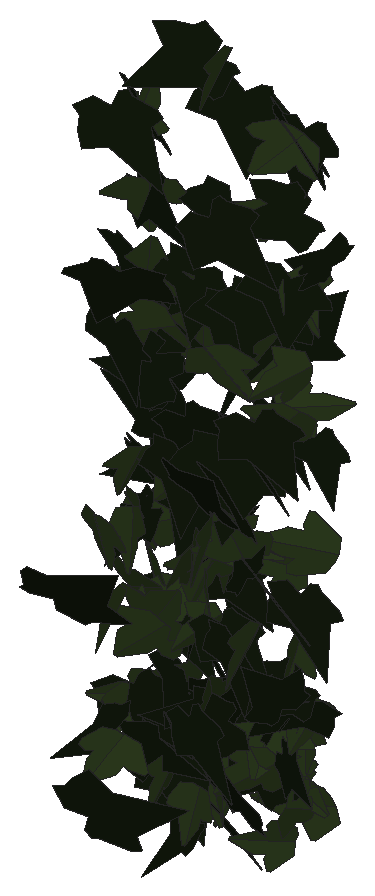
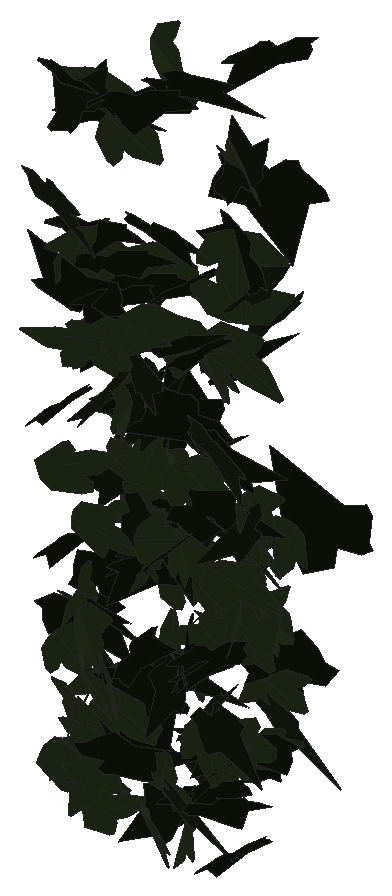
# SketchUp Ruby script. Lengths in inches.
U = 1.inch
M = Sketchup.active_model
def pt(a) = Geom::Point3d.new(a.map { |v| v * U })
def face(e, loops, mat)
  f = e.add_face(loops[0].map { |a| pt(a) })
  loops[1..].each { |l| e.add_face(l.map { |a| pt(a) }).erase! }
  f.material = f.back_material = mat if mat
  f
end
# faces: each face lists its corners as indices into pts; further lists are holes
def faces(e, pts, list, mat = nil) = list.each { |f| face(e, (f[0].is_a?(Array) ? f : [f]).map { |l| l.map { |i| pts[i] } }, mat) }
# xy, xz, yz: faces in a plane at the given z, y or x. An outline is a flat list of corners, or four numbers for a rectangle; further outlines are holes
def ring(l) = l.size == 4 ? [[l[0], l[1]], [l[2], l[1]], [l[2], l[3]], [l[0], l[3]]] : l.each_slice(2).to_a
def flat(e, list, mat, &to3) = list.each { |f| face(e, (f[0].is_a?(Array) ? f : [f]).map { |l| ring(l).map { |u, v| to3.(u, v) } }, mat) }
def xy(e, z, list, mat = nil) = flat(e, list, mat) { |x, y| [x, y, z] }
def xz(e, y, list, mat = nil) = flat(e, list, mat) { |x, z| [x, y, z] }
def yz(e, x, list, mat = nil) = flat(e, list, mat) { |y, z| [x, y, z] }
def lines(e, pts, list) = list.each { |a, b| e.add_line(pt(pts[a]), pt(pts[b])) }
# prism: a flat outline (further loops are holes) pulled along v
def prism(e, loops, v, mat = nil)
  f = face(e, loops, mat); d = Geom::Vector3d.new(v.map { |x| x * U })
  f.pushpull(f.normal.samedirection?(d) ? d.length : -d.length)
end
def box(e, o, s, mat = nil) = prism(e, [[o, [o[0] + s[0], o[1], o[2]], [o[0] + s[0], o[1] + s[1], o[2]], [o[0], o[1] + s[1], o[2]]]], [0, 0, s[2]], mat)
def at(x, y, z, deg = 0) = Geom::Transformation.translation(pt([x, y, z])) * Geom::Transformation.rotation(ORIGIN, Z_AXIS, deg.degrees)
def axes(o, x, y, z) = Geom::Transformation.new([*x, 0, *y, 0, *z, 0, *pt(o).to_a, 1])
def part(name) = M.definitions.add(name)
# library, detail: a bought-in or finely detailed component or shape, given as its bounding box
def library(name, o, s) = part(name).tap { |d| box(d.entities, o, s) }
def detail(e, o, s) = box(e.add_group.entities, o, s)
def put(e, d, t, mat = nil) = e.add_instance(d, t).tap { |i| i.material = mat if mat }
def group(e, t, mat = nil) = e.add_group.tap { |g| g.transformation = t; g.material = mat if mat }.entities
root = M.entities
M.materials.add("1026 AP 7946 SUNNY SIDE UP").color = [254, 231, 186]
M.materials.add("efeu1").color = [18, 25, 13]
M.materials.add("efeu2").color = [43, 57, 29]
c1 = part("ivyleaf_9")
p = [[1.54,2.16,1.25],[1.36,2.04,1.19],[-0.21,0.99,0.68],[-0.71,1.11,0.82],[-0.85,0.86,0.67],[-0.8,0.17,0.21],
  [-0.9,-0.01,0.1],[-0.67,-0.16,-0.02],[-0.08,-0.08,-0.05],[-0.03,-0.6,-0.4],[0.65,-0.88,-0.66],[0.83,-0.6,-0.49],
  [1.29,-0.42,-0.43],[1.8125,-0.07,-0.26],[1.21,0.44,0.15]]
faces(c1.entities,p,[[0,1,2,3,4,5,6,7,8,9,10,11,12,13,14]],"efeu1")
c2 = part("ivyleaf_10")
p = [[0,0.5,-0.03],[-0.0625,2.02,-0.43],[-0.19,2.01,-0.46],[-0.54,1.05,-0.29],[-0.52,0.625,-0.18],[-0.83,0.76,-0.28],
  [-1.16,0.64,-0.33],[-1.15,0.33,-0.24],[-0.77,-0.39,0.02],[-0.3,-0.51,0.16],[0.04,-0.48,0.23],[-0.02,2.01,-0.4375],
  [-0.06,2.01,-0.43],[0.04,-0.49,0.23],[0.67,-0.49,0.14],[1.38,0.36,-0.2],[1.375,0.51,-0.24],[0.81,0.65,-0.19],
  [0.62,0.59,-0.15],[0.6,1.09,-0.28],[0.5,1.23,-0.31]]
faces(c2.entities,p,[[0,1,2,3,4,5,6,7,8,9,10],[11,12,0,13,14,15,16,17,18,19,20]],"efeu2")
put(root,c1,axes([122.75,208.77,268.89],[0.03474,0.02424,0.377],[0.53606,-0.13615,-0.01271],[0.21202,0.34025,-0.02963]),"1026 AP 7946 SUNNY SIDE UP")
put(root,c1,axes([121.66,209.41,271.47],[0.60179,0.0809,-0.03944],[0.04372,0.05444,0.40035],[0.1341,-0.38081,0.04648]),"1026 AP 7946 SUNNY SIDE UP")
put(root,c2,axes([123.75,209.64,269.13],[0.39833,-0.15611,0.07489],[0.07791,-0.05941,-0.3059],[0.25994,0.25702,-0.02308]),"1026 AP 7946 SUNNY SIDE UP")
put(root,c2,axes([122.36,209.76,269.38],[0.30396,0.15864,-0.17189],[-0.1758,-0.12711,-0.2573],[-0.31765,0.22216,-0.02208]),"1026 AP 7946 SUNNY SIDE UP")
put(root,c1,axes([122.5,209.63,276.52],[0.28706,0.22973,-0.2263],[-0.18683,-0.18725,-0.30277],[-0.46509,0.21701,-0.01805]),"1026 AP 7946 SUNNY SIDE UP")
put(root,c1,axes([123.41,210.02,269.98],[0.19558,-0.3098,-0.09677],[-0.07178,0.08094,-0.34322],[0.50313,0.13197,-0.01135]),"1026 AP 7946 SUNNY SIDE UP")
put(root,c2,axes([124.22,210.21,271.46],[0.09418,-0.28362,0.22119],[0.1015,-0.2071,-0.29937],[0.55161,0.08653,0.01732]),"1026 AP 7946 SUNNY SIDE UP")
put(root,c1,axes([122.08,210.05,278.63],[0.03794,-0.29954,-0.21207],[0.02738,0.20533,-0.30704],[0.56934,0.01009,0.0289]),"1026 AP 7946 SUNNY SIDE UP")
put(root,c1,axes([121.99,210.16,269.31],[-0.37422,0.23918,-0.03857],[0.01295,-0.04637,-0.34678],[-0.38078,-0.23663,0.02612]),"1026 AP 7946 SUNNY SIDE UP")
put(root,c1,axes([123.23,210.27,268.25],[-0.37725,0.13435,-0.15103],[0.16463,-0.11135,-0.28083],[-0.26688,-0.25861,0.04026]),"1026 AP 7946 SUNNY SIDE UP")
put(root,c1,axes([123.67,210.13,277.5],[0.10698,-0.22666,-0.28735],[-0.03255,0.27964,-0.23878],[0.56263,0.05928,0.04082]),"1026 AP 7946 SUNNY SIDE UP")
put(root,c1,axes([123.8,210.43,271.08],[0.02352,-0.30816,0.07438],[0.00007,-0.07403,-0.31825],[0.49831,0.01455,-0.00346]),"1026 AP 7946 SUNNY SIDE UP")
put(root,c2,axes([123.31,210.48,272.58],[0.16811,-0.25804,0.21936],[0.15013,-0.19231,-0.28862],[0.5057,0.14287,0.01277]),"1026 AP 7946 SUNNY SIDE UP")
put(root,c1,axes([123.08,210.46,273.07],[0.49405,-0.12793,-0.06342],[0.1154,0.02041,0.3464],[-0.19052,-0.31938,0.04537]),"1026 AP 7946 SUNNY SIDE UP")
put(root,c1,axes([124.52,210.48,270.39],[0.10657,0.0934,0.29273],[-0.36115,-0.16955,0.11307],[0.30005,-0.23725,0.03212]),"1026 AP 7946 SUNNY SIDE UP")
put(root,c1,axes([121.72,210.57,275.05],[0.07536,-0.34041,0.10363],[0.03011,-0.10083,-0.3547],[0.5582,0.0514,0.00514]),"1026 AP 7946 SUNNY SIDE UP")
put(root,c2,axes([121.71,210.59,270.93],[0.10354,-0.24939,0.23301],[0.12107,-0.21469,-0.26655],[0.51691,0.10024,0.01575]),"1026 AP 7946 SUNNY SIDE UP")
put(root,c1,axes([124.1,210.55,272.1],[0.28603,-0.21039,0.12753],[0.09847,-0.11053,-0.28621],[0.37197,0.19103,-0.0223]),"1026 AP 7946 SUNNY SIDE UP")
put(root,c2,axes([123.47,210.42,275.27],[-0.39701,-0.06742,-0.16391],[0.25675,-0.00295,-0.26632],[0.08722,-0.29822,0.03785]),"1026 AP 7946 SUNNY SIDE UP")
put(root,c1,axes([123.57,210.46,271.27],[0.09627,-0.26634,-0.16801],[0.04134,0.1685,-0.27488],[0.48808,0.03826,0.05642]),"1026 AP 7946 SUNNY SIDE UP")
put(root,c2,axes([121.53,210.45,272.08],[-0.39499,0.15912,-0.01322],[-0.00242,-0.02801,-0.30546],[-0.25111,-0.25001,0.02374]),"1026 AP 7946 SUNNY SIDE UP")
put(root,c2,axes([123.1,210.78,271.05],[-0.04722,-0.11263,0.28485],[0.00635,-0.27867,-0.11785],[0.47035,-0.00755,0.03019]),"1026 AP 7946 SUNNY SIDE UP")
put(root,c2,axes([122.4375,210.74,268.65],[0.02735,-0.23179,0.2053],[0.10044,-0.19377,-0.2375],[0.47142,0.05473,0.03869]),"1026 AP 7946 SUNNY SIDE UP")
put(root,c2,axes([124.51,210.83,275.23],[-0.04906,-0.07801,0.33838],[-0.01486,-0.32997,-0.08348],[0.53131,-0.01643,0.02891]),"1026 AP 7946 SUNNY SIDE UP")
put(root,c2,axes([122.96,210.52,272.14],[0.05841,-0.33956,-0.1479],[0.01997,0.14346,-0.35003],[0.57817,0.02935,0.02703]),"1026 AP 7946 SUNNY SIDE UP")
put(root,c2,axes([123.68,210.68,272.35],[-0.37359,-0.19004,-0.13045],[-0.18168,-0.05578,0.31192],[-0.30864,0.26287,-0.02571]),"1026 AP 7946 SUNNY SIDE UP")
put(root,c2,axes([122.32,210.65,270.69],[-0.37508,-0.07457,0.21036],[-0.27563,-0.11435,-0.25412],[0.20321,-0.29274,0.0436]),"1026 AP 7946 SUNNY SIDE UP")
put(root,c1,axes([123.44,210.67,269.71],[-0.09254,-0.08527,-0.29251],[-0.36862,-0.16301,0.09971],[-0.28415,0.23924,-0.03409]),"1026 AP 7946 SUNNY SIDE UP")
put(root,c1,axes([123.62,210.74,272.9],[0.18318,-0.30368,0.05041],[0.00472,0.05528,0.33461],[-0.48409,-0.11437,0.02234]),"1026 AP 7946 SUNNY SIDE UP")
put(root,c1,axes([121.92,210.58,268.94],[0.17731,-0.03785,-0.27747],[0.3614,0.16876,0.07575],[0.22804,-0.23804,0.0957]),"1026 AP 7946 SUNNY SIDE UP")
put(root,c1,axes([122.3,210.86,274.35],[-0.13919,-0.0046,0.32221],[-0.37911,-0.20612,-0.07462],[0.31341,-0.25137,0.05284]),"1026 AP 7946 SUNNY SIDE UP")
put(root,c1,axes([123.97,210.65,274.31],[-0.07011,-0.23844,-0.23444],[0.0656,0.22234,-0.2486],[0.51263,-0.06106,-0.00025]),"1026 AP 7946 SUNNY SIDE UP")
put(root,c2,axes([121.74,210.8,272.07],[0.35308,-0.15175,0.17713],[0.20708,-0.11313,-0.27932],[0.29644,0.25977,-0.01585]),"1026 AP 7946 SUNNY SIDE UP")
put(root,c2,axes([123.15,210.83,269.9],[-0.07626,-0.24225,-0.17779],[-0.01191,-0.17241,0.25252],[-0.46629,0.04402,0.02263]),"1026 AP 7946 SUNNY SIDE UP")
put(root,c2,axes([122.27,210.6875,270.83],[-0.45804,0.02765,0.14058],[0.21745,0.02403,0.29959],[0.02319,0.32071,-0.03267]),"1026 AP 7946 SUNNY SIDE UP")
put(root,c1,axes([123.59,210.76,268.43],[0.2861,-0.22137,0.17389],[-0.1302,0.15105,0.29473],[-0.41918,-0.19801,0.02714]),"1026 AP 7946 SUNNY SIDE UP")
put(root,c2,axes([123.85,210.92,277.28],[-0.14352,-0.24233,0.24192],[-0.06436,-0.23494,-0.26598],[0.5282,-0.09447,0.03332]),"1026 AP 7946 SUNNY SIDE UP")
put(root,c1,axes([122.49,210.99,273.1],[-0.0741,-0.33047,0.06776],[-0.00702,-0.06769,-0.34425],[0.53036,-0.04707,0.00491]),"1026 AP 7946 SUNNY SIDE UP")
put(root,c2,axes([123.02,210.87,271.88],[-0.22661,-0.2897,0.08494],[-0.02272,-0.08647,-0.33287],[0.47379,-0.14271,0.02467]),"1026 AP 7946 SUNNY SIDE UP")
put(root,c2,axes([122.78,210.94,271.51],[0.18814,-0.09722,0.26448],[0.32824,-0.15059,-0.15951],[0.28159,0.24049,0.00923]),"1026 AP 7946 SUNNY SIDE UP")
put(root,c1,axes([123.38,210.97,273.47],[-0.38306,-0.26247,-0.11254],[0.15474,0.05503,-0.36701],[0.41844,-0.26063,0.0327]),"1026 AP 7946 SUNNY SIDE UP")
put(root,c1,axes([123.86,210.59,272.06],[-0.02057,0.17138,0.2591],[-0.05711,0.24808,-0.17533],[-0.47386,-0.03734,0.00988]),"1026 AP 7946 SUNNY SIDE UP")
put(root,c1,axes([121.7,211.1,275.7],[-0.19087,-0.17255,0.29828],[0.07881,-0.31448,-0.17268],[0.52543,-0.01551,0.13426]),"1026 AP 7946 SUNNY SIDE UP")
put(root,c2,axes([121.625,210.98,269.28],[0.17107,0.19239,-0.21146],[-0.15826,-0.18015,-0.22874],[-0.41443,0.14821,0.00006]),"1026 AP 7946 SUNNY SIDE UP")
put(root,c1,axes([124.55,210.91,270.27],[0.10137,0.09592,-0.27197],[-0.1958,-0.23366,-0.11991],[-0.3968,0.1398,-0.01031]),"1026 AP 7946 SUNNY SIDE UP")
put(root,c2,axes([123.89,211,269.06],[-0.22355,-0.17079,0.25958],[-0.21762,-0.21262,-0.22929],[0.42772,-0.19744,0.01901]),"1026 AP 7946 SUNNY SIDE UP")
put(root,c1,axes([124.36,211.07,277.43],[-0.39822,-0.08811,0.15737],[-0.20903,-0.08159,-0.2751],[0.18324,-0.28456,0.02819]),"1026 AP 7946 SUNNY SIDE UP")
put(root,c1,axes([121.92,210.99,272.18],[-0.39726,0.10747,-0.15529],[0.20031,-0.08553,-0.28214],[-0.21229,-0.28181,0.02437]),"1026 AP 7946 SUNNY SIDE UP")
put(root,c1,axes([124.35,211.02,270.4],[-0.45268,-0.00458,-0.00237],[0.00427,-0.02796,-0.29538],[0.00683,-0.28654,0.02717]),"1026 AP 7946 SUNNY SIDE UP")
put(root,c2,axes([123.89,211.15,275.17],[0.0814,0.14518,-0.27014],[-0.18009,-0.23723,-0.15949],[-0.43675,0.12488,0.01542]),"1026 AP 7946 SUNNY SIDE UP")
put(root,c2,axes([124.17,211.1,274.29],[-0.26732,-0.21932,0.18705],[-0.15334,-0.15538,-0.28636],[0.42196,-0.19541,0.01444]),"1026 AP 7946 SUNNY SIDE UP")
put(root,c1,axes([123.3,211.15,273.69],[0.27411,-0.27955,0.11365],[0.07239,-0.10304,-0.33967],[0.46791,0.17971,-0.01403]),"1026 AP 7946 SUNNY SIDE UP")
put(root,c2,axes([121.77,211.22,269.3],[0.01176,-0.01126,-0.34528],[-0.38739,-0.22754,0.00088],[-0.3576,0.24612,-0.01231]),"1026 AP 7946 SUNNY SIDE UP")
put(root,c1,axes([124.2,210.96,269.3125],[0.21303,-0.16307,-0.2014],[-0.23021,0.12998,-0.21649],[0.32611,0.19828,-0.02127]),"1026 AP 7946 SUNNY SIDE UP")
put(root,c2,axes([121.48,211.15,272.01],[0.09631,-0.05982,0.28966],[0.40217,-0.12065,-0.08444],[0.20748,0.26162,0.02923]),"1026 AP 7946 SUNNY SIDE UP")
put(root,c2,axes([121.82,211.07,275.5],[-0.45849,-0.2308,-0.00255],[-0.02607,0.01908,0.38233],[-0.36198,0.29096,-0.02431]),"1026 AP 7946 SUNNY SIDE UP")
put(root,c1,axes([122.31,211.12,268.49],[-0.07859,-0.30708,-0.1281],[0.05647,0.11822,-0.31944],[0.51685,-0.05961,0.01542]),"1026 AP 7946 SUNNY SIDE UP")
put(root,c2,axes([121.54,211.15,270.83],[-0.35197,0.04121,0.28142],[0.39732,-0.11087,0.23008],[0.17473,0.33513,0.04371]),"1026 AP 7946 SUNNY SIDE UP")
put(root,c2,axes([121.5625,211.15,272.81],[-0.06852,-0.27852,0.07641],[0.00193,-0.07679,-0.29058],[0.45385,-0.04172,0.01277]),"1026 AP 7946 SUNNY SIDE UP")
put(root,c1,axes([122.23,211.35,269.57],[-0.08708,-0.23252,0.25782],[-0.03983,-0.25137,-0.24655],[0.53719,-0.05633,0.02351]),"1026 AP 7946 SUNNY SIDE UP")
put(root,c2,axes([123.82,211.14,269.61],[0.32513,0.27611,-0.11778],[-0.09217,-0.1008,-0.35571],[-0.46174,0.21454,-0.01193]),"1026 AP 7946 SUNNY SIDE UP")
put(root,c1,axes([121.66,211.03,269.44],[-0.11734,-0.15189,-0.29739],[0.20881,0.25537,-0.17282],[0.46718,-0.15229,0.00254]),"1026 AP 7946 SUNNY SIDE UP")
put(root,c2,axes([122.5,211.2,272.94],[-0.29222,-0.19324,0.18795],[-0.17215,-0.14865,-0.2763],[0.38207,-0.21477,0.01926]),"1026 AP 7946 SUNNY SIDE UP")
put(root,c1,axes([123.21,211.25,275.48],[-0.27125,-0.24196,-0.04674],[0.0624,0.02565,-0.30547],[0.38163,-0.17617,0.01672]),"1026 AP 7946 SUNNY SIDE UP")
put(root,c2,axes([122.67,211.13,271.85],[-0.02743,-0.35177,-0.01727],[-0.00184,0.01484,-0.36275],[0.55361,-0.01738,-0.00206]),"1026 AP 7946 SUNNY SIDE UP")
put(root,c2,axes([124.51,211.31,272.35],[0.01859,0.12449,0.33171],[-0.22195,-0.29151,0.12001],[0.49424,-0.13559,0.04142]),"1026 AP 7946 SUNNY SIDE UP")
put(root,c2,axes([122.05,211.14,274.9],[-0.31421,-0.01255,0.31255],[-0.46336,-0.07992,-0.20378],[0.11561,-0.35444,0.0327]),"1026 AP 7946 SUNNY SIDE UP")
put(root,c1,axes([122.51,211.08,273.71],[-0.03968,-0.04157,-0.3235],[0.37685,0.2031,-0.04639],[0.3251,-0.24051,0.01429]),"1026 AP 7946 SUNNY SIDE UP")
put(root,c1,axes([122.89,211.11,268.03],[0.39139,-0.13194,-0.02807],[-0.05446,-0.00896,-0.28922],[0.20448,0.25016,-0.02329]),"1026 AP 7946 SUNNY SIDE UP")
put(root,c1,axes([123.03,211.02,271.92],[-0.07178,0.29615,-0.02521],[-0.00218,-0.02667,-0.3088],[-0.46748,-0.04535,0.00531]),"1026 AP 7946 SUNNY SIDE UP")
put(root,c2,axes([122.67,211.28,268.33],[0.23768,-0.05363,0.28148],[0.35482,-0.15913,-0.16153],[0.2573,0.26897,-0.03726]),"1026 AP 7946 SUNNY SIDE UP")
put(root,c1,axes([122.85,211.07,269.67],[0.2325,0.00705,0.24802],[0.37642,-0.03492,-0.15065],[0.04103,0.28033,-0.02334]),"1026 AP 7946 SUNNY SIDE UP")
put(root,c1,axes([124.07,210.93,269.72],[0.01006,0.14305,0.25703],[-0.02575,0.24852,-0.14538],[-0.45037,-0.01101,0.01406]),"1026 AP 7946 SUNNY SIDE UP")
put(root,c2,axes([124.16,211.34,270.77],[0.01582,0.20605,-0.27357],[-0.04314,-0.26545,-0.21388],[-0.5282,0.02785,0.00927]),"1026 AP 7946 SUNNY SIDE UP")
put(root,c2,axes([124.42,211.31,269.94],[-0.16833,-0.23603,0.17079],[0.01762,-0.18146,-0.25768],[0.45441,-0.0804,0.07326]),"1026 AP 7946 SUNNY SIDE UP")
put(root,c2,axes([123.87,211.35,267.76],[-0.02382,-0.03377,-0.29634],[-0.3201,-0.20338,0.03448],[-0.32352,0.20372,-0.0123]),"1026 AP 7946 SUNNY SIDE UP")
put(root,c1,axes([123.65,211.36,275.68],[-0.32801,-0.28131,-0.03082],[0.05483,0.00933,-0.36],[0.44118,-0.21031,0.02182]),"1026 AP 7946 SUNNY SIDE UP")
put(root,c1,axes([122.43,211.4,275.74],[-0.11508,-0.31017,0.07119],[-0.01494,-0.07055,-0.32865],[0.50006,-0.07349,0.00656]),"1026 AP 7946 SUNNY SIDE UP")
put(root,c1,axes([124.21,211.31,271.54],[0.03053,-0.33821,-0.07417],[-0.01339,0.0697,-0.34856],[0.54294,0.02074,-0.00443]),"1026 AP 7946 SUNNY SIDE UP")
put(root,c1,axes([122.48,211.33,272.47],[-0.38942,-0.10747,-0.13027],[0.20759,0.00826,-0.27489],[0.1569,-0.27767,0.04037]),"1026 AP 7946 SUNNY SIDE UP")
put(root,c2,axes([122.14,211.33,270.92],[0.34615,0.14305,-0.13777],[-0.14946,-0.09925,-0.2695],[-0.2702,0.23815,-0.02742]),"1026 AP 7946 SUNNY SIDE UP")
put(root,c2,axes([123.14,211.09,272.19],[0.1007,0.09092,0.28403],[0.26195,0.21907,-0.11323],[-0.37291,0.17844,-0.00284]),"1026 AP 7946 SUNNY SIDE UP")
put(root,c2,axes([122.77,211.45,279.01],[0.12029,-0.27053,0.19004],[0.08667,-0.17769,-0.29064],[0.5089,0.09421,0.00458]),"1026 AP 7946 SUNNY SIDE UP")
put(root,c2,axes([123.91,211.43,269.61],[0.33236,-0.20171,0.1772],[0.1659,-0.1394,-0.30079],[0.38368,0.23501,-0.02345]),"1026 AP 7946 SUNNY SIDE UP")
put(root,c2,axes([122.0625,211.35,274.76],[0.38665,-0.16337,0.0215],[0.00821,-0.0314,-0.30338],[0.25902,0.24486,-0.02247]),"1026 AP 7946 SUNNY SIDE UP")
put(root,c1,axes([123.6,211.19,268.55],[-0.32712,0.18872,0.17555],[0.21545,-0.10062,0.28836],[0.33545,0.24866,-0.01401]),"1026 AP 7946 SUNNY SIDE UP")
put(root,c1,axes([123.92,211.43,276.1],[-0.30109,-0.20731,-0.11646],[0.1594,0.05761,-0.28842],[0.33436,-0.21415,0.03263]),"1026 AP 7946 SUNNY SIDE UP")
put(root,c2,axes([121.79,211.42,271.81],[-0.22037,-0.05069,0.26795],[-0.30586,-0.1806,-0.14513],[0.28362,-0.23415,0.05168]),"1026 AP 7946 SUNNY SIDE UP")
put(root,c2,axes([122.6,211.32,275.02],[-0.45808,-0.07175,0.02266],[-0.02302,-0.03381,-0.30782],[0.11593,-0.29022,0.02843]),"1026 AP 7946 SUNNY SIDE UP")
put(root,c1,axes([122.45,211.55,274.94],[-0.33345,-0.15933,0.15773],[-0.15157,-0.12562,-0.27135],[0.31375,-0.23002,0.03655]),"1026 AP 7946 SUNNY SIDE UP")
put(root,c1,axes([122.3,211.52,270.7],[-0.03074,-0.02174,-0.30262],[0.36924,-0.17867,-0.00352],[-0.27928,-0.23383,0.02865]),"1026 AP 7946 SUNNY SIDE UP")
put(root,c2,axes([124.19,211.13,268.5],[-0.04601,-0.14367,-0.2956],[0.15372,0.26958,-0.14817],[0.47938,-0.10023,0.01915]),"1026 AP 7946 SUNNY SIDE UP")
put(root,c1,axes([121.89,211.38,269],[0.09907,-0.27436,-0.08424],[-0.03821,0.0767,-0.28948],[0.44783,0.06724,-0.00607]),"1026 AP 7946 SUNNY SIDE UP")
put(root,c1,axes([122.16,211.49,272.73],[-0.07736,-0.04658,-0.30204],[-0.18943,-0.26819,0.06321],[-0.42617,0.12766,0.02673]),"1026 AP 7946 SUNNY SIDE UP")
put(root,c1,axes([122.98,211.32,271.55],[-0.03221,-0.19298,-0.22795],[0.05906,0.21716,-0.19841],[0.45656,-0.04171,0.00958]),"1026 AP 7946 SUNNY SIDE UP")
put(root,c1,axes([121.36,211.62,277.67],[-0.048,-0.14233,0.33211],[0.10317,-0.32102,-0.14114],[0.5456,0.04819,0.05591]),"1026 AP 7946 SUNNY SIDE UP")
put(root,c2,axes([121.7,211.32,271.3],[-0.26338,0.23814,0.03146],[-0.05859,0.00934,-0.29878],[-0.37268,-0.16977,0.02474]),"1026 AP 7946 SUNNY SIDE UP")
put(root,c1,axes([123.16,211.53,272.29],[-0.21686,0.07594,-0.24353],[0.22576,-0.19681,-0.1523],[-0.31931,-0.19072,0.05771]),"1026 AP 7946 SUNNY SIDE UP")
put(root,c1,axes([121.97,211.31,273.38],[-0.0997,0.07021,0.28935],[-0.34693,0.17381,-0.0952],[-0.2938,-0.22907,0.01422]),"1026 AP 7946 SUNNY SIDE UP")
put(root,c2,axes([123.79,211.32,269.83],[0.15922,-0.24553,-0.16001],[-0.10759,0.13818,-0.27264],[0.44279,0.12187,-0.00871]),"1026 AP 7946 SUNNY SIDE UP")
put(root,c2,axes([123.34,211.45,273.72],[-0.22597,0.2335,-0.13741],[0.07847,-0.12697,-0.28232],[-0.41655,-0.15059,0.02136]),"1026 AP 7946 SUNNY SIDE UP")
put(root,c2,axes([123.92,211.46,278.18],[0.45462,-0.03116,-0.15382],[-0.2376,-0.0178,-0.29807],[0.03059,0.32483,-0.02917]),"1026 AP 7946 SUNNY SIDE UP")
put(root,c1,axes([121.33,211.54,276.63],[0.04148,-0.09499,-0.33355],[0.52974,0.0084,0.02583],[0.00158,-0.3242,0.09634]),"1026 AP 7946 SUNNY SIDE UP")
put(root,c1,axes([122.02,211.42,270.5],[0.0823,-0.26384,-0.15151],[-0.00882,0.14687,-0.27545],[0.47373,0.04857,0.02119]),"1026 AP 7946 SUNNY SIDE UP")
put(root,c2,axes([122.01,211.47,269.59],[-0.19682,-0.31352,0.00848],[0.01252,-0.01395,-0.34762],[0.49308,-0.12479,0.01221]),"1026 AP 7946 SUNNY SIDE UP")
put(root,c2,axes([123.94,211.48,270.45],[0.02845,-0.31297,0.01203],[0.00013,-0.01347,-0.32304],[0.49257,0.01808,-0.00061]),"1026 AP 7946 SUNNY SIDE UP")
put(root,c2,axes([124.05,211.31,274.34],[0.09971,-0.01757,-0.30478],[0.40698,0.15046,0.04884],[0.2267,-0.26239,0.04637]),"1026 AP 7946 SUNNY SIDE UP")
put(root,c1,axes([123.04,211.63,274.46],[-0.25208,0.01335,-0.26342],[0.32333,-0.17318,-0.1431],[-0.24009,-0.24724,0.08385]),"1026 AP 7946 SUNNY SIDE UP")
put(root,c2,axes([123.9,211.4375,271.85],[0.0921,-0.04965,-0.31898],[-0.47082,0.08379,-0.07177],[0.14505,0.3035,-0.03041]),"1026 AP 7946 SUNNY SIDE UP")
put(root,c2,axes([124.32,211.5,268.4],[0.15214,-0.01136,-0.32216],[-0.49087,0.01799,-0.1001],[0.03231,0.32678,-0.00377]),"1026 AP 7946 SUNNY SIDE UP")
put(root,c2,axes([121.54,211.48,276.65],[-0.39673,-0.22602,-0.00557],[0.03053,-0.01551,-0.34815],[0.35414,-0.25187,0.02377]),"1026 AP 7946 SUNNY SIDE UP")
put(root,c1,axes([121.32,211.47,272.6875],[0.36269,-0.17941,-0.0554],[-0.05917,0.03753,-0.30075],[0.28804,0.23362,0.00798]),"1026 AP 7946 SUNNY SIDE UP")
put(root,c2,axes([122.97,211.28,271.72],[0.07825,-0.14832,-0.28963],[0.07779,0.28388,-0.14404],[0.49254,-0.02127,0.06876]),"1026 AP 7946 SUNNY SIDE UP")
put(root,c2,axes([123.7,211.44,268.74],[0.27435,0.08349,0.25915],[0.37372,0.08273,-0.198],[-0.18286,0.29434,-0.01586]),"1026 AP 7946 SUNNY SIDE UP")
put(root,c1,axes([123.41,211.53,275.33],[-0.04788,-0.26521,-0.14317],[0.06008,0.13359,-0.27344],[0.46585,-0.04448,0.02055]),"1026 AP 7946 SUNNY SIDE UP")
put(root,c2,axes([122.46,211.3,267.96],[0.03367,-0.11271,-0.2798],[-0.01332,0.27133,-0.11538],[0.46125,0.01606,0.01709]),"1026 AP 7946 SUNNY SIDE UP")
put(root,c2,axes([122.81,211.42,268.55],[0.50368,-0.04397,0.10962],[-0.15747,0.05025,0.3315],[-0.09004,-0.33386,0.03343]),"1026 AP 7946 SUNNY SIDE UP")
put(root,c1,axes([121.86,211.51,269.82],[-0.19591,0.24077,-0.11565],[0.0445,-0.11276,-0.27879],[-0.41625,-0.12537,0.02462]),"1026 AP 7946 SUNNY SIDE UP")
put(root,c1,axes([122.54,211.45,270.11],[0.36218,-0.10674,-0.15468],[-0.23105,0.03694,-0.26011],[0.17343,0.27213,-0.0235]),"1026 AP 7946 SUNNY SIDE UP")
put(root,c2,axes([121.38,211.47,277.59],[0.41065,-0.21004,0.03028],[-0.00211,0.04686,0.34359],[-0.33375,-0.25873,0.03509]),"1026 AP 7946 SUNNY SIDE UP")
put(root,c1,axes([123.46,211.64,273.92],[0.20983,-0.2938,-0.02156],[-0.03294,0.01162,-0.33203],[0.46178,0.13433,-0.01388]),"1026 AP 7946 SUNNY SIDE UP")
put(root,c1,axes([122.36,211.72,278.79],[-0.48598,-0.08088,0.1262],[-0.17397,-0.06093,-0.32813],[0.15262,-0.327,0.02783]),"1026 AP 7946 SUNNY SIDE UP")
put(root,c2,axes([123.93,211.64,269.38],[0.39062,-0.09166,0.13126],[0.17984,-0.05908,-0.27274],[0.16999,0.27311,-0.01309]),"1026 AP 7946 SUNNY SIDE UP")
put(root,c1,axes([123.95,211.69,278.24],[-0.34015,-0.09573,-0.2197],[0.35332,-0.00762,-0.23193],[0.09849,-0.3033,0.07322]),"1026 AP 7946 SUNNY SIDE UP")
put(root,c2,axes([122.8,211.49,275.16],[-0.27638,-0.18781,-0.15839],[0.217,0.07724,-0.26111],[0.31265,-0.21963,0.04122]),"1026 AP 7946 SUNNY SIDE UP")
put(root,c1,axes([121.86,211.58,270.81],[-0.02079,-0.26023,-0.1765],[-0.00297,0.17007,-0.26729],[0.48862,-0.01004,-0.00913]),"1026 AP 7946 SUNNY SIDE UP")
put(root,c2,axes([122.78,211.64,268.09],[0.29569,-0.2268,0.0236],[0.00211,-0.03026,-0.30311],[0.35864,0.18717,-0.01768]),"1026 AP 7946 SUNNY SIDE UP")
put(root,c1,axes([121.4,211.71,268.17],[-0.01118,-0.3108,-0.02862],[0.00863,0.0259,-0.32007],[0.49033,-0.00754,0.00498]),"1026 AP 7946 SUNNY SIDE UP")
put(root,c1,axes([122.01,211.72,275.07],[-0.04224,-0.29439,-0.00878],[-0.00016,0.00689,-0.30449],[0.46302,-0.02685,-0.00091]),"1026 AP 7946 SUNNY SIDE UP")
put(root,c2,axes([122.69,211.82,272.2],[0.00998,-0.08098,0.29469],[0.05033,-0.28473,-0.0853],[0.46545,0.03252,0.0029]),"1026 AP 7946 SUNNY SIDE UP")
put(root,c1,axes([122.45,211.72,272.08],[0.08676,-0.27462,-0.02592],[-0.01842,0.02171,-0.28835],[0.43302,0.05595,-0.00707]),"1026 AP 7946 SUNNY SIDE UP")
put(root,c1,axes([122.9,211.75,278.39],[-0.2439,-0.29261,-0.10979],[0.08982,0.08841,-0.34054],[0.48045,-0.16507,0.00793]),"1026 AP 7946 SUNNY SIDE UP")
put(root,c1,axes([123.37,211.73,268.81],[-0.1607,0.06287,0.32408],[-0.50386,-0.02355,-0.10265],[0.00535,-0.32959,0.06715]),"1026 AP 7946 SUNNY SIDE UP")
put(root,c2,axes([123.93,211.55,275.97],[0.05549,0.32588,0.10135],[0.02518,0.09535,-0.33708],[-0.53383,0.03837,-0.00537]),"1026 AP 7946 SUNNY SIDE UP")
put(root,c1,axes([122.625,211.78,276.66],[-0.43769,-0.06867,-0.09406],[0.15292,-0.01819,-0.29271],[0.09332,-0.29226,0.03851]),"1026 AP 7946 SUNNY SIDE UP")
put(root,c1,axes([123.66,211.9,278.03],[0.07601,-0.24786,0.26944],[0.13965,-0.24901,-0.26008],[0.55077,0.09734,0.02876]),"1026 AP 7946 SUNNY SIDE UP")
put(root,c1,axes([123.83,211.625,275.13],[-0.2721,0.08946,0.27911],[0.37903,-0.12257,0.19997],[0.2386,0.29673,0.00065]),"1026 AP 7946 SUNNY SIDE UP")
put(root,c1,axes([121.59,211.85,268.85],[-0.28213,-0.23309,0.00311],[0.01779,-0.01418,-0.30257],[0.36614,-0.17892,0.0171]),"1026 AP 7946 SUNNY SIDE UP")
put(root,c1,axes([124.08,211.8,273.66],[0.0274,-0.29711,-0.0166],[-0.01641,0.01383,-0.30637],[0.46745,0.0179,-0.00978]),"1026 AP 7946 SUNNY SIDE UP")
put(root,c1,axes([124.47,211.56,276.48],[-0.19115,0.26388,0.09551],[-0.10485,0.06917,-0.29728],[-0.42631,-0.13533,0.03029]),"1026 AP 7946 SUNNY SIDE UP")
put(root,c1,axes([121.88,211.5,273.72],[-0.1002,0.26608,0.16218],[-0.0997,0.1445,-0.27991],[-0.47457,-0.08654,0.02456]),"1026 AP 7946 SUNNY SIDE UP")
put(root,c1,axes([122.33,211.74,268.69],[-0.38459,0.17286,-0.07745],[0.07283,-0.06592,-0.30775],[-0.28795,-0.24755,0.02561]),"1026 AP 7946 SUNNY SIDE UP")
put(root,c2,axes([123.7,211.63,268.51],[-0.19589,-0.2327,-0.1457],[0.12872,0.11481,-0.27076],[0.40725,-0.14822,0.0155]),"1026 AP 7946 SUNNY SIDE UP")
put(root,c1,axes([122.8125,211.95,270.6],[0.01324,-0.07286,-0.29001],[0.19764,-0.25259,0.06985],[-0.41162,-0.12362,0.02421]),"1026 AP 7946 SUNNY SIDE UP")
